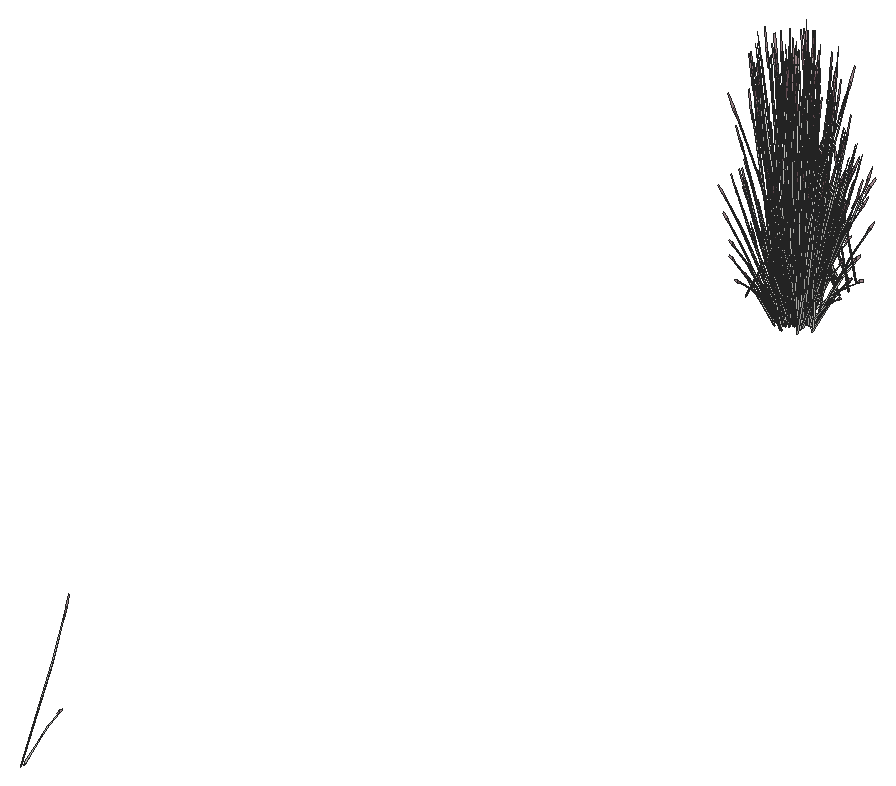
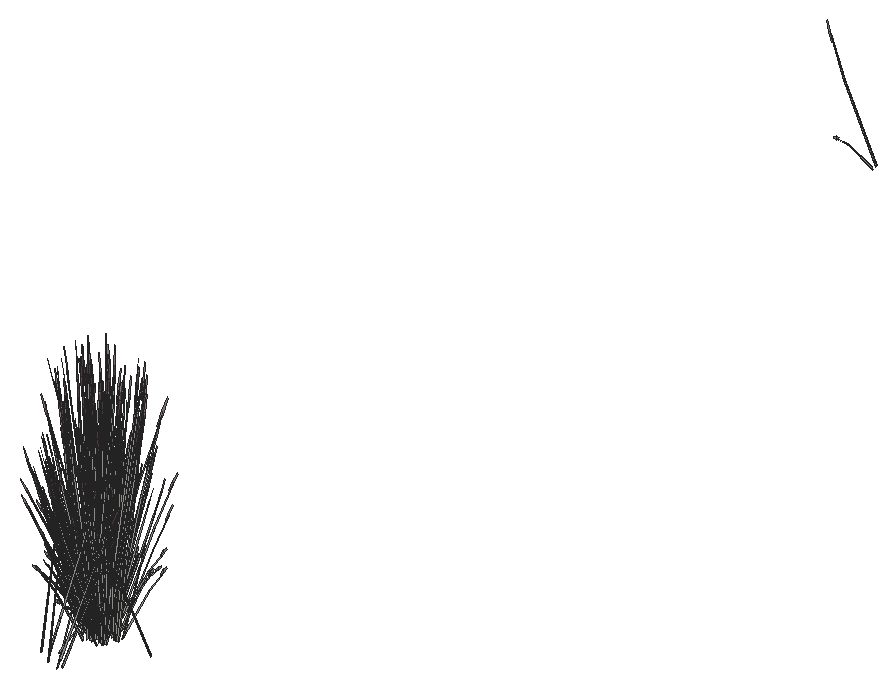
# SketchUp Ruby script. Lengths in inches.
U = 1.inch
M = Sketchup.active_model
def pt(a) = Geom::Point3d.new(a.map { |v| v * U })
def face(e, loops, mat)
  f = e.add_face(loops[0].map { |a| pt(a) })
  loops[1..].each { |l| e.add_face(l.map { |a| pt(a) }).erase! }
  f.material = f.back_material = mat if mat
  f
end
# faces: each face lists its corners as indices into pts; further lists are holes
def faces(e, pts, list, mat = nil) = list.each { |f| face(e, (f[0].is_a?(Array) ? f : [f]).map { |l| l.map { |i| pts[i] } }, mat) }
# xy, xz, yz: faces in a plane at the given z, y or x. An outline is a flat list of corners, or four numbers for a rectangle; further outlines are holes
def ring(l) = l.size == 4 ? [[l[0], l[1]], [l[2], l[1]], [l[2], l[3]], [l[0], l[3]]] : l.each_slice(2).to_a
def flat(e, list, mat, &to3) = list.each { |f| face(e, (f[0].is_a?(Array) ? f : [f]).map { |l| ring(l).map { |u, v| to3.(u, v) } }, mat) }
def xy(e, z, list, mat = nil) = flat(e, list, mat) { |x, y| [x, y, z] }
def xz(e, y, list, mat = nil) = flat(e, list, mat) { |x, z| [x, y, z] }
def yz(e, x, list, mat = nil) = flat(e, list, mat) { |y, z| [x, y, z] }
def lines(e, pts, list) = list.each { |a, b| e.add_line(pt(pts[a]), pt(pts[b])) }
# prism: a flat outline (further loops are holes) pulled along v
def prism(e, loops, v, mat = nil)
  f = face(e, loops, mat); d = Geom::Vector3d.new(v.map { |x| x * U })
  f.pushpull(f.normal.samedirection?(d) ? d.length : -d.length)
end
def box(e, o, s, mat = nil) = prism(e, [[o, [o[0] + s[0], o[1], o[2]], [o[0] + s[0], o[1] + s[1], o[2]], [o[0], o[1] + s[1], o[2]]]], [0, 0, s[2]], mat)
def at(x, y, z, deg = 0) = Geom::Transformation.translation(pt([x, y, z])) * Geom::Transformation.rotation(ORIGIN, Z_AXIS, deg.degrees)
def axes(o, x, y, z) = Geom::Transformation.new([*x, 0, *y, 0, *z, 0, *pt(o).to_a, 1])
def part(name) = M.definitions.add(name)
# library, detail: a bought-in or finely detailed component or shape, given as its bounding box
def library(name, o, s) = part(name).tap { |d| box(d.entities, o, s) }
def detail(e, o, s) = box(e.add_group.entities, o, s)
def put(e, d, t, mat = nil) = e.add_instance(d, t).tap { |i| i.material = mat if mat }
def group(e, t, mat = nil) = e.add_group.tap { |g| g.transformation = t; g.material = mat if mat }.entities
root = M.entities
M.materials.add("LightPink_Translucent").color = [144, 107, 117]
M.materials["LightPink_Translucent"].alpha = 0.75
c1 = part("blade")
p = [[2.15,0.21,22],[0,0.17,0],[0.09,0.45,0],[2.18,0.31,22],[2.29,0.31,22],[0.38,0.45,0],
  [2.48,0.24,33],[2.49,0.24,33],[2.48,0.22,33]]
faces(c1.entities,p,[[0,1,2,3],[4,5,2,3],[6,3,4,7],[8,0,3,6]])
c2 = part("seeds")
p = [[0.3,-0.1,1.38],[-0.01,-0.03,1.59],[-0.01,-0.03,0.03],[0.14,-0.07,-0.07],[0.29,-0.03,3],[0.15,0.01,3.11]]
faces(c2.entities,p,[[0,1,2,3],[1,0,4,5]],"LightPink_Translucent")
c3 = part("blade with seeds")
put(c3.entities,c1,at(0,0,0))
put(c3.entities,c2,axes([2.4,0.25,30.99],[1.5799,-0.05474,1.17369],[-0.12525,1.92788,0.29478],[-0.07173,-0.02425,1.56792]))
put(root,c3,axes([505.97,212.85,4.17],[0.36264,0.49684,-0.71045],[-0.74649,0.27689,0.08574],[0.0848,0.24006,1.00501]))
put(root,c3,axes([505.43,214.1,3.91],[0.09631,0.0984,1.74944],[0.77725,0.03866,-0.27667],[0.07816,0.217,0.14031]))
put(root,c3,axes([507.97,440.58,3.07],[0.17368,0.19618,1.71376],[-0.80256,0.16516,0.13857],[-0.18139,-0.30799,0.73262]))
put(root,c3,axes([509.3,439.28,3.91],[-0.11621,-0.08567,1.74944],[-0.77555,0.05431,-0.27667],[-0.12378,-0.20491,0.14031]))
put(root,c3,axes([511.1,440.3,1.78],[-0.21597,0.12368,1.43002],[-0.64681,-0.21647,-0.30754],[0.1199,-0.26922,0.61141]))
put(root,c3,axes([510.11,440.73,4.17],[-0.36264,-0.49684,-0.71045],[0.74649,-0.27689,0.08574],[-0.0848,-0.24006,1.00501]))
put(root,c3,axes([507.75,440.0625,1.78],[-0.04601,0.19989,1.43002],[-0.67263,0.16733,-0.30754],[-0.15723,-0.25836,0.61141]))
put(root,c3,axes([509.49,439.625,0.6875],[-0.12744,0.02202,1.76342],[-0.70477,-0.24781,-0.26939],[0.01183,-0.2067,0.30037]))
put(root,c3,axes([511.625,441.21,4.17],[0.01977,-0.56521,-0.71045],[0.83252,0.03796,0.08574],[0.08786,-0.23945,1.00501]))
put(root,c3,axes([512.78,440.33,3.91],[-0.00733,-0.12161,1.74944],[-0.61946,-0.35147,-0.27667],[0.09577,-0.21306,0.14031]))
put(root,c3,axes([510.18,440.31,3.72],[0.22906,-0.4699,-0.35414],[0.66828,0.13705,0.4572],[-0.06128,-0.18919,0.87481]))
put(root,c3,axes([510.6875,440.93,3.07],[-0.14147,0.21002,1.71376],[-0.59349,-0.43464,0.13857],[0.26773,-0.27089,0.73262]))
put(root,c3,axes([512.62,439.89,3.9],[-0.07716,0.04667,1.77383],[-0.75601,-0.15746,-0.16761],[-0.02737,-0.20368,0.31391]))
put(root,c3,axes([509.84,440.63,3.875],[-0.7469,-0.15318,-0.51099],[0.25601,-0.52518,-0.3958],[-0.06849,-0.21144,0.97773]))
put(root,c3,axes([510.3,439.3125,1.96],[0.09747,0.35631,1.1486],[-0.54071,-0.19735,0.84392],[0.05818,-0.18244,0.25299]))
put(root,c3,axes([511.45,441.03,3.875],[-0.54391,-0.41056,-0.51099],[0.57458,-0.35956,-0.3958],[0.08276,-0.2086,0.97773]))
put(root,c3,axes([508.5,439,3.9],[-0.01417,0.07324,1.77383],[-0.6991,0.2658,-0.16761],[-0.20573,-0.13587,0.31391]))
put(root,c3,axes([508.35,440.3,4.29],[0.84639,-0.15705,0.53763],[0.14689,0.61608,0.4433],[-0.19906,-0.18157,1.11249]))
put(root,c3,axes([510.26,440.41,3.93],[0.74868,0.15974,0.48003],[-0.25601,0.52518,0.3958],[-0.04499,-0.20653,0.9933]))
put(root,c3,axes([510.48,440.6,4.23],[-0.74352,0.28449,-0.1216],[-0.36538,-0.50492,-0.67495],[-0.0981,-0.21277,1.02557]))
put(root,c3,axes([512.02,441.24,4.23],[-0.83505,-0.03027,-0.1216],[0.02282,-0.57322,-0.67495],[0.05801,-0.22077,1.02557]))
put(root,c3,axes([511.97,440.875,3.72],[0.5141,-0.32171,-0.35414],[0.48666,0.36734,0.4572],[0.07405,-0.18664,0.87481]))
put(root,c3,axes([507.52,439.74,1.96],[0.39634,0.21267,1.1486],[-0.57721,0.12784,0.84392],[-0.1235,-0.16344,0.25299]))
put(root,c3,axes([510.46,440.375,3.92],[0.55987,-0.20767,0.0643],[0.27403,0.37869,0.50621],[-0.05407,-0.16693,0.77189]))
put(root,c3,axes([508.26,440.48,3.72],[-0.11735,-0.49217,-0.35414],[0.67083,-0.12996,0.4572],[-0.18018,-0.14104,0.87481]))
put(root,c3,axes([508.55,440.43,3.92],[0.34533,-0.38816,0.0643],[0.49176,0.22599,0.50621],[-0.15898,-0.12445,0.77189]))
put(root,c3,axes([507.21,440.38,0.6875],[-0.0736,0.08049,1.76342],[-0.74378,0.17355,-0.26939],[-0.17968,-0.15788,0.30037]))
put(root,c3,axes([508.4375,442.59,1.29],[-0.31203,-0.62659,-0.69835],[0.89884,-0.22566,-0.18329],[-0.03449,-0.21218,1.54149]))
put(root,c3,axes([512.61,440.68,0.6875],[-0.11372,-0.04814,1.76342],[-0.29211,-0.53779,-0.26939],[0.19706,-0.14594,0.30037]))
put(root,c3,axes([510.26,440.8,4.24],[-0.22906,0.4699,0.35414],[-0.66828,-0.13705,-0.4572],[-0.06128,-0.18919,0.87481]))
put(root,c3,axes([511.96,441,3.93],[0.54105,0.41691,0.48003],[-0.57458,0.35956,0.3958],[0.0998,-0.1956,0.9933]))
put(root,c3,axes([512.16,441.04,3.92],[0.62439,0.02847,0.0643],[-0.01712,0.42991,0.50621],[0.06534,-0.16468,0.77189]))
put(root,c3,axes([511.7,441.33,4.24],[-0.5141,0.32171,0.35414],[-0.48666,-0.36734,-0.4572],[0.07405,-0.18664,0.87481]))
put(root,c3,axes([512.6,442.2,4.17],[0.39688,-0.48213,-0.71045],[0.69548,0.34264,0.08574],[0.23697,-0.17468,1.00501]))
put(root,c3,axes([508.3125,440.79,1.57],[-0.47504,-0.61229,0],[0.79476,-0.34146,-0.51607],[0.18101,-0.07777,1.63711]))
put(root,c3,axes([512.58,441.97,3.875],[-0.19519,-0.55794,-0.51099],[0.73919,-0.0976,-0.3958],[0.21183,-0.14986,0.97773]))
put(root,c3,axes([509.36,440.05,1.32],[-0.52505,0.35054,-0.03893],[-0.48109,-0.38392,-0.17649],[-0.03387,-0.10878,0.58215]))
put(root,c3,axes([512.93,442.37,4.23],[-0.70283,-0.33692,-0.1216],[0.40491,-0.48793,-0.67495],[0.19857,-0.16961,1.02557]))
put(root,c3,axes([510.03,444.21,2.52],[0.65659,0.2464,1.51261],[-0.64324,0.53082,0.59816],[-0.28812,-0.31461,1.26806]))
put(root,c3,axes([508.65,440.88,4.24],[0.11735,0.49217,0.35414],[-0.67083,0.12996,-0.4572],[-0.18018,-0.14104,0.87481]))
put(root,c3,axes([506.6,442.51,1.21],[0,-0.61104,-0.49651],[0.85008,0,0],[0,-0.13917,1.57504]))
put(root,c3,axes([508.96,440.7,1.21],[0.7111,-0.30552,-0.49651],[0.42504,0.54784,0],[0.16196,-0.06958,1.57504]))
put(root,c3,axes([513.18,441.75,1.78],[-0.27143,-0.0181,1.43002],[-0.27808,-0.48551,-0.30754],[0.33346,-0.13735,0.61141]))
put(root,c3,axes([514.66,442.22,3.9],[-0.09924,-0.00464,1.77383],[-0.4121,-0.49725,-0.16761],[0.1655,-0.1635,0.31391]))
put(root,c3,axes([509.8,441.95,1.25],[0.51177,-0.45928,-0.62353],[0.63575,0.41646,-0.16365],[0.20507,-0.11457,1.37633]))
put(root,c3,axes([513.49,440.86,1.96],[-0.25308,0.31105,1.1486],[-0.21753,-0.4179,0.84392],[0.20902,-0.10472,0.25299]))
put(root,c3,axes([513.13,442.03,3.72],[0.66138,-0.08733,-0.35414],[0.17464,0.49921,0.4572],[0.18953,-0.13408,0.87481]))
put(root,c3,axes([508.91,442.76,1.4],[0.36864,-0.55059,-0.44739],[0.76598,0.26498,0.21531],[0,-0.12692,1.43643]))
put(root,c3,axes([509.25,442.48,1.86],[-0.08854,-0.69723,-0.29095],[0.92215,-0.04216,-0.50002],[0.16238,-0.09287,1.59708]))
put(root,c3,axes([506.96,442.52,1.22],[0.53038,-0.38124,-0.30978],[0.53038,0.38124,0.30978],[0,-0.1228,1.38974]))
put(root,c3,axes([506.75,440.69,1.32],[-0.21918,0.49894,-0.03893],[-0.6746,-0.15348,-0.17649],[-0.10242,-0.08161,0.58215]))
put(root,c3,axes([512.59,442.32,4.24],[-0.66138,0.08733,0.35414],[-0.17464,-0.49921,-0.4572],[0.18953,-0.13408,0.87481]))
put(root,c3,axes([508.82,443.21,1.86],[-0.85568,-0.29155,-0.29095],[0.41201,-0.61537,-0.50002],[-0.02689,-0.15109,1.59708]))
put(root,c3,axes([506.38,442.97,1.57],[-0.95008,0,0],[0,-0.68292,-0.51607],[0,-0.15554,1.63711]))
put(root,c3,axes([509.125,440.9375,1.22],[0.70886,0.15119,-0.30978],[-0.17848,0.53243,0.30978],[0.1429,-0.0614,1.38974]))
put(root,c3,axes([513.19,442.25,3.92],[0.52161,0.25698,0.0643],[-0.30368,0.36595,0.50621],[0.16723,-0.11831,0.77189]))
put(root,c3,axes([513.04,442.14,3.93],[0.18844,0.56237,0.48003],[-0.73919,0.0976,0.3958],[0.21785,-0.13226,0.9933]))
put(root,c3,axes([515.04,442.82,3.91],[0.10543,-0.09307,1.74944],[-0.13495,-0.57092,-0.27667],[0.26455,-0.10825,0.14031]))
put(root,c3,axes([507.12,442.79,1.52],[-0.70674,0.51372,0.30756],[-0.70717,-0.50832,-0.36492],[-0.02468,-0.14589,1.64885]))
put(root,c3,axes([509.37,443.03,1.625],[0.8561,0.29616,0.24065],[-0.41201,0.61537,0.50002],[0,-0.14185,1.60543]))
put(root,c3,axes([509.03,443.86,1.63],[0.20138,-0.72405,-0.23429],[0.95485,0.12621,0.51271],[-0.16685,-0.09999,1.5644]))
put(root,c3,axes([509.09,442.62,1.91],[-0.82508,0.03772,0.44739],[-0.07462,-0.62614,-0.21531],[0.14771,-0.06346,1.43643]))
put(root,c3,axes([506.96,443.07,1.67],[0,0.61104,0.49651],[-0.85008,0,0],[0,-0.13917,1.57504]))
put(root,c3,axes([512.96,443.69,4.23],[-0.38229,-0.5533,-0.1216],[0.6785,-0.2719,-0.67495],[0.28593,-0.073,1.02557]))
put(root,c3,axes([512.93,443.21,3.875],[0.20584,-0.55581,-0.51099],[0.70573,0.19051,-0.3958],[0.28414,-0.05097,0.97773]))
put(root,c3,axes([511.8125,440.95,1.57],[0.47504,-0.61229,0],[0.79476,0.34146,-0.51607],[0.18101,0.07777,1.63711]))
put(root,c3,axes([508.97,443.57,1.4],[-0.45644,-0.51287,-0.44739],[0.69137,-0.36116,0.21531],[-0.14771,-0.06346,1.43643]))
put(root,c3,axes([509.0625,442.84,1.55],[0.33034,0.68327,0.45755],[-0.94388,0.2376,0.17955],[0.01154,-0.12555,1.58856]))
put(root,c3,axes([513.68,443.37,1.17],[-0.48937,0.07333,1.41583],[-0.07789,-0.58369,0.08104],[0.34275,-0.08835,0.80566]))
put(root,c3,axes([514.57,442.85,1.45],[-0.47106,-0.39072,-0.06488],[0.51591,-0.35801,-0.29416],[0.14618,-0.02521,0.97024]))
put(root,c3,axes([508.9,443.38,1.91],[-0.36864,0.55059,0.44739],[-0.76598,-0.26498,-0.21531],[0,-0.12692,1.43643]))
put(root,c3,axes([510.25,442.9,1.4],[0,-0.70701,0],[0.95008,0,0],[0,0,1.79456]))
put(root,c3,axes([511.4,441.27,1.67],[-0.7111,-0.30552,0.49651],[0.42504,-0.54784,0],[0.16196,0.06958,1.57504]))
put(root,c3,axes([512.79,443.41,4.17],[0.66765,-0.26986,-0.71045],[0.37208,0.55551,0.08574],[0.32259,-0.0631,1.00501]))
put(root,c3,axes([509.8,442.45,1.55],[-0.62999,0.55453,0.45755],[-0.74845,-0.4895,0.17955],[0.15188,-0.05534,1.58856]))
put(root,c3,axes([510.49,443.45,1.49],[-0.70674,-0.52593,-0.06131],[0.70717,-0.52625,0],[-0.02468,-0.01837,1.75571]))
put(root,c3,axes([508.71,441.54,1.67],[-0.21949,0.60727,0.17642],[-0.8032,-0.17185,0.35086],[0.13875,-0.00296,1.60407]))
put(root,c3,axes([512.7,443.52,4.24],[-0.63144,-0.17046,0.35414],[0.18417,-0.49731,-0.4572],[0.25423,-0.0456,0.87481]))
put(root,c3,axes([508.375,442.03,0.79],[-0.74787,0.24464,1.28929],[-0.23804,-0.70192,0.50096],[0.45924,0.01168,1.46642]))
put(root,c3,axes([510.38,442.22,1.81],[0.14658,-0.54532,0.1448],[0.71613,0.09466,-0.41347],[0.13033,0.05599,1.26744]))
put(root,c3,axes([509.15,443.51,1.55],[0.96033,0.12874,0.45755],[-0.19544,0.7271,0.17955],[-0.14034,-0.07021,1.58856]))
put(root,c3,axes([514.22,442.98,0.6875],[-0.03971,-0.09277,1.76342],[0.27541,-0.54264,-0.26939],[0.27782,-0.00781,0.30037]))
put(root,c3,axes([510.08,442.36,1.91],[-0.45644,-0.51287,0.44739],[0.69137,-0.36116,-0.21531],[0.14771,0.06346,1.43643]))
put(root,c3,axes([507.72,444.7,1.22],[-0.17848,-0.53243,-0.30978],[0.70886,-0.15119,0.30978],[-0.1429,-0.0614,1.38974]))
put(root,c3,axes([508.63,444.67,1.67],[0.81646,-0.16218,0.17642],[0.20161,0.60355,0.35086],[-0.07282,-0.08794,1.60407]))
put(root,c3,axes([510.3125,442.39,1.86],[0.76714,-0.40567,-0.29095],[0.51013,0.57321,-0.50002],[0.18927,0.05821,1.59708]))
put(root,c3,axes([513.36,443.46,3.72],[0.63144,0.17046,-0.35414],[-0.18417,0.49731,0.4572],[0.25423,-0.0456,0.87481]))
put(root,c3,axes([507.52,444.93,1.21],[-0.7111,-0.30552,-0.49651],[0.42504,-0.54784,0],[-0.16196,-0.06958,1.57504]))
put(root,c3,axes([512.24,441.32,1.21],[0.7111,0.30552,-0.49651],[-0.42504,0.54784,0],[0.16196,0.06958,1.57504]))
put(root,c3,axes([510.9,443.06,1.4],[0.85008,0,0],[0,0.63259,0],[0,0,1.78407]))
put(root,c3,axes([509.45,443.85,1.86],[-0.76714,0.40567,-0.29095],[-0.51013,-0.57321,-0.50002],[-0.18927,-0.05821,1.59708]))
put(root,c3,axes([511.14,441.57,1.67],[-0.81646,0.16218,0.17642],[-0.20161,-0.60355,0.35086],[0.07282,0.08794,1.60407]))
put(root,c3,axes([511.64,442.85,3.07],[-0.31515,0.01384,1.71376],[0.20907,-0.5998,0.13857],[0.44912,0.0371,0.73262]))
put(root,c3,axes([512.05,441.54,1.22],[0.17848,0.53243,-0.30978],[-0.70886,0.15119,0.30978],[0.1429,0.0614,1.38974]))
put(root,c3,axes([513.27,443.67,3.92],[0.27906,0.41663,0.0643],[-0.50888,0.20393,0.50621],[0.22432,-0.04024,0.77189]))
put(root,c3,axes([510.62,442.74,1.57],[-0.96033,-0.12874,0.49198],[0.19544,-0.7271,0.19306],[0.14034,0.07021,1.70813]))
put(root,c3,axes([513.21,443.52,3.93],[-0.21466,0.55714,0.48003],[-0.70573,-0.19051,0.3958],[0.27753,-0.03348,0.9933]))
put(root,c3,axes([509.86,444.53,1.4],[-0.24791,-0.5268,0],[0.70791,-0.18448,0],[0,0,1.54371]))
put(root,c3,axes([509.38,444.03,1.81],[-0.14658,0.54532,0.1448],[-0.71613,-0.09466,-0.41347],[-0.13033,-0.05599,1.26744]))
put(root,c3,axes([510.78,444.46,1.38],[0.79769,-0.20732,-0.19198],[0.2803,0.59721,0.00008],[0.08805,-0.02292,1.73897]))
put(root,c3,axes([511.06,444.71,1.67],[0.21949,-0.60727,0.17642],[0.8032,0.17185,0.35086],[-0.13875,0.00296,1.60407]))
put(root,c3,axes([510.875,443.33,1.41],[0.53038,0.39469,0],[-0.53038,0.39469,0],[0,0,1.69266]))
put(root,c3,axes([512.3125,443.16,1.67],[-0.59697,-0.44509,0.17642],[0.60159,-0.4317,0.35086],[-0.06593,0.0909,1.60407]))
put(root,c3,axes([511.21,442.49,1.25],[0.79037,0.10018,-0.62353],[-0.16679,0.61794,-0.16365],[0.23587,0.07488,1.37633]))
put(root,c3,axes([514.7,443.56,1.96],[-0.46945,0.10088,1.1486],[0.22097,-0.4169,0.84392],[0.24904,0.02853,0.25299]))
put(root,c3,axes([509.68,444.77,1.39],[-0.76598,-0.27433,0],[0.36864,-0.57001,0],[0,0,1.62707]))
put(root,c3,axes([510.32,444.04,1.66],[-0.74193,-0.49181,-0.25192],[0.6243,-0.55226,0.5513],[-0.19979,0.05753,1.68216]))
put(root,c3,axes([508.36,444.98,1.67],[0.7111,0.30552,0.49651],[-0.42504,0.54784,0],[-0.16196,-0.06958,1.57504]))
put(root,c3,axes([510.87,442.87,1.91],[0.36864,-0.55059,0.44739],[0.76598,0.26498,-0.21531],[0,0.12692,1.43643]))
put(root,c3,axes([514.48,445.33,3.9],[-0.0687,-0.05349,1.77383],[0.15029,-0.57341,-0.16761],[0.27062,-0.03664,0.31391]))
put(root,c3,axes([510.73,443.18,1.48],[0,0.70667,-0.05637],[-0.95008,0,0],[0,0.02221,1.79368]))
put(root,c3,axes([510.8,442.68,1.4],[0.45644,0.51287,-0.44739],[-0.69137,0.36116,0.21531],[0.14771,0.06346,1.43643]))
put(root,c3,axes([513.88,444.85,3.12],[-0.14542,-0.51365,-0.03492],[0.68734,-0.11809,-0.15832],[0.14353,0.03256,0.52218]))
put(root,c3,axes([507.95,445.3,1.57],[-0.47504,0.61229,0],[-0.79476,-0.34146,-0.51607],[-0.18101,-0.07777,1.63711]))
put(root,c3,axes([512.1,444.83,4.23],[0.04068,-0.62141,-0.1216],[0.77029,0.01698,-0.67495],[0.29667,0.04317,1.02557]))
put(root,c3,axes([512.8,443.17,1.67],[0,-0.61104,0.49651],[0.85008,0,0],[0,0.13917,1.57504]))
put(root,c3,axes([510.67,443.63,1.91],[0.82508,-0.03772,0.44739],[0.07462,0.62614,-0.21531],[-0.14771,0.06346,1.43643]))
put(root,c3,axes([511.19,442.99,1.81],[0.70791,-0.1782,0.1448],[0.24791,0.50885,-0.41347],[0,0.11199,1.26744]))
put(root,c3,axes([511.98,444.59,4.24],[-0.43232,-0.38257,0.35414],[0.49364,-0.36215,-0.4572],[0.25081,0.0551,0.87481]))
put(root,c3,axes([509.94,443.94,1.4],[-0.82508,0.03772,-0.44739],[-0.07462,-0.62614,0.21531],[-0.14771,0.06346,1.43643]))
put(root,c3,axes([497.11,444.23,1.78],[-0.18299,-0.15028,1.43002],[0.23809,-0.49714,-0.30754],[0.37023,0.06735,0.61141]))
put(root,c3,axes([513.82,444.23,1.78],[-0.18299,-0.15028,1.43002],[0.23809,-0.49714,-0.30754],[0.37023,0.06735,0.61141]))
put(root,c3,axes([510.55,444.78,1.4],[0.76598,0.27433,0],[-0.36864,0.57001,0],[0,0,1.74954]))
put(root,c3,axes([512.77,444.46,3.91],[0.16299,-0.01033,1.74944],[0.44707,-0.47471,-0.27667],[0.28992,0.06266,0.14031]))
put(root,c3,axes([510.85,445.39,1.39],[-0.46912,-0.61443,-0.05142],[0.79476,-0.34146,0.51607],[-0.19584,0.0585,1.6363]))
put(root,c3,axes([510.6875,443.9,1.81],[0.56134,0.36712,0.1448],[-0.46823,0.41419,-0.41347],[-0.13033,0.05599,1.26744]))
put(root,c3,axes([512.14,444.54,4.17],[0.75952,0.01471,-0.71045],[-0.05101,0.61953,0.08574],[0.32177,0.06538,1.00501]))
put(root,c3,axes([511.29,445.03,1.67],[0.7111,-0.30552,0.49651],[0.42504,0.54784,0],[-0.16196,0.06958,1.57504]))
put(root,c3,axes([510.27,444.55,1.48],[0.33034,0.70197,-0.06012],[-0.94388,0.24598,0],[0.01154,0.02451,1.72173]))
put(root,c3,axes([510.64,445.31,1.22],[-0.70886,-0.15119,-0.30978],[0.17848,-0.53243,0.30978],[-0.1429,0.0614,1.38974]))
put(root,c3,axes([506.71,443.81,4.24],[0.66138,-0.08733,0.35414],[0.17464,0.49921,-0.4572],[-0.18953,0.13408,0.87481]))
put(root,c3,axes([513.38,443.28,1.57],[0.95008,0,0],[0,0.68292,-0.51607],[0,0.15554,1.63711]))
put(root,c3,axes([513,443.63,1.39],[-0.94962,-0.00489,-0.04976],[0,-0.68292,0.49943],[-0.02984,0.15546,1.58352]))
put(root,c3,axes([510.95,443.03,1.86],[0.85568,0.29155,-0.29095],[-0.41201,0.61537,-0.50002],[0.02689,0.15109,1.59708]))
put(root,c3,axes([512.6,444.79,3.72],[0.43232,0.38257,-0.35414],[-0.49364,0.36215,0.4572],[0.25081,0.0551,0.87481]))
put(root,c3,axes([512.8,443.73,1.22],[-0.53038,0.38124,-0.30978],[-0.53038,-0.38124,0.30978],[0,0.1228,1.38974]))
put(root,c3,axes([510.52,443.77,1.86],[0.08854,0.69723,-0.29095],[-0.92215,0.04216,-0.50002],[-0.16238,0.09287,1.59708]))
put(root,c3,axes([512.375,444.9375,3.92],[-0.03826,0.46465,0.0643],[-0.57772,-0.01274,0.50621],[0.2213,0.04862,0.77189]))
put(root,c3,axes([510.86,443.49,1.4],[-0.36864,0.55059,-0.44739],[-0.76598,-0.26498,0.21531],[0,0.12692,1.43643]))
put(root,c3,axes([512.43,444.79,3.93],[-0.56024,0.40262,0.48003],[-0.48318,-0.42758,0.3958],[0.26285,0.07427,0.9933]))
put(root,c3,axes([505.21,445.23,4.84],[0.67048,0.16311,-0.06488],[-0.20625,0.50201,-0.29416],[-0.10966,0.07622,0.97024]))
put(root,c3,axes([509.96,444.3,1.25],[-0.51177,0.45928,-0.62353],[-0.63575,-0.41646,-0.16365],[-0.20507,0.11457,1.37633]))
put(root,c3,axes([510.65,445.26,4.24],[-0.11735,-0.49217,0.35414],[0.67083,-0.12996,-0.4572],[0.18018,0.14104,0.87481]))
put(root,c3,axes([510.875,445.07,1.52],[0.95122,0.19861,0.30756],[-0.23797,0.7099,-0.36492],[-0.15744,0.08885,1.64885]))
put(root,c3,axes([510.81,445.55,1.21],[-0.7111,0.30552,-0.49651],[-0.42504,-0.54784,0],[-0.16196,0.06958,1.57504]))
put(root,c3,axes([513.17,443.74,1.21],[0,0.61104,-0.49651],[-0.85008,0,0],[0,0.13917,1.57504]))
put(root,c3,axes([511.04,443.81,3.07],[-0.28223,-0.10528,1.71376],[0.58406,-0.44165,0.13857],[0.36402,0.19924,0.73262]))
put(root,c3,axes([511.1,442.42,3.67],[-0.65655,-0.31748,1.38283],[0.69326,-0.49431,0.59665],[0.21183,0.29789,1.33663]))
put(root,c3,axes([506.37,443.76,4.23],[0.70283,0.33692,-0.1216],[-0.40491,0.48793,-0.67495],[-0.19857,0.16961,1.02557]))
put(root,c3,axes([512.09,445.01,1.96],[-0.4278,-0.1757,1.1486],[0.5524,-0.17852,0.84392],[0.14899,0.15122,0.25299]))
put(root,c3,axes([510.59,445.51,4.23],[0.45276,-0.52302,-0.1216],[0.65568,0.30132,-0.67495],[0.22792,0.14777,1.02557]))
put(root,c3,axes([507.6,444.8,4.24],[0.5141,-0.32171,0.35414],[0.48666,0.36734,-0.4572],[-0.07405,0.18664,0.87481]))
put(root,c3,axes([511.45,445.46,1.57],[0.47504,0.61229,0],[-0.79476,0.34146,-0.51607],[-0.18101,0.07777,1.63711]))
put(root,c3,axes([509.99,445.94,3.9],[0.00225,-0.07398,1.77383],[0.65113,-0.32638,-0.16761],[0.22617,0.1165,0.31391]))
put(root,c3,axes([512.21,445.66,0.6875],[0.05536,-0.08822,1.76342],[0.69692,-0.25981,-0.26939],[0.21129,0.13447,0.30037]))
put(root,c3,axes([511.05,443.03,2.03],[-0.02076,-0.57531,1.41272],[0.93937,0.14913,0.59816],[-0.22217,0.31481,1.3335]))
put(root,c3,axes([511.29,443.66,1.29],[0.2786,0.55945,-0.69212],[-0.80253,0.20149,-0.18165],[0.03079,0.18945,1.52773]))
put(root,c3,axes([507.14,445.1,3.92],[-0.62439,-0.02847,0.0643],[0.01712,-0.42991,0.50621],[-0.06534,0.16468,0.77189]))
put(root,c3,axes([507.33,445.14,3.93],[-0.54105,-0.41691,0.48003],[0.57458,-0.35956,0.3958],[-0.0998,0.1956,0.9933]))
put(root,c3,axes([511.12,445.25,3.875],[0.74975,-0.14525,-0.51099],[0.13115,0.55007,-0.3958],[0.20138,0.15763,0.97773]))
put(root,c3,axes([509.04,445.33,4.24],[0.22906,-0.4699,0.35414],[0.66828,0.13705,-0.4572],[0.06128,0.18919,0.87481]))
put(root,c3,axes([512.16,445.81,1.86],[-0.48723,-0.01916,1.0506],[0.32177,-0.40701,0.58006],[0.19248,0.1446,0.8241]))
put(root,c3,axes([510.75,445.7,3.92],[-0.34533,0.38816,0.0643],[-0.49176,-0.22599,0.50621],[0.15898,0.12445,0.77189]))
put(root,c3,axes([509.94,447.01,4.84],[0.52505,-0.35054,-0.06488],[0.48109,0.38392,-0.29416],[0.03387,0.10878,0.97024]))
put(root,c3,axes([510.9,445.59,3.93],[-0.75571,0.14023,0.48003],[-0.13115,-0.55007,0.3958],[0.17773,0.16212,0.9933]))
put(root,c3,axes([510.57,444.82,1.78],[0.01341,-0.20255,1.43002],[0.64074,-0.22625,-0.30754],[0.1978,0.24243,0.61141]))
put(root,c3,axes([508.84,445.76,3.92],[-0.55987,0.20767,0.0643],[-0.27403,-0.37869,0.50621],[0.05407,0.16693,0.77189]))
put(root,c3,axes([507.33,445.26,3.72],[-0.5141,0.32171,-0.35414],[-0.48666,-0.36734,0.4572],[-0.07405,0.18664,0.87481]))
put(root,c3,axes([507.27,444.89,4.59],[0.83505,0.03027,-0.13498],[-0.02282,0.57322,-0.74919],[-0.05801,0.22077,1.13838]))
put(root,c3,axes([508.82,445.53,4.23],[0.74352,-0.28449,-0.1216],[0.36538,0.50492,-0.67495],[0.0981,0.21277,1.02557]))
put(root,c3,axes([509.03,445.72,4.26],[-0.74868,-0.15974,0.53283],[0.25601,-0.52518,0.43934],[0.04499,0.20653,1.10256]))
put(root,c3,axes([507.66,446.51,1.96],[-0.01966,-0.36332,1.1486],[0.49135,0.25914,0.84392],[-0.09663,0.17317,0.25299]))
put(root,c3,axes([508.95,445.64,0.6875],[0.12297,-0.03325,1.76342],[0.73967,0.18301,-0.26939],[0.02163,0.20626,0.30037]))
put(root,c3,axes([507.84,445.11,4.2],[0.54391,0.41056,-0.5672],[-0.57458,0.35956,-0.43934],[-0.08276,0.2086,1.08528]))
put(root,c3,axes([507.25,445.73,2.02],[0.69024,-0.1082,0.06507],[0.15868,0.43593,-0.86304],[-0.04376,0.22067,0.7736]))
put(root,c3,axes([509.46,445.51,3.875],[0.7469,0.15318,-0.51099],[-0.25601,0.52518,-0.3958],[0.06849,0.21144,0.97773]))
put(root,c3,axes([509.88,444.42,3.07],[-0.17368,-0.19618,1.71376],[0.80256,-0.16516,0.13857],[0.18139,0.30799,0.73262]))
put(root,c3,axes([509.12,445.83,3.72],[-0.22906,0.4699,-0.35414],[-0.66828,-0.13705,0.4572],[0.06128,0.18919,0.87481]))
put(root,c3,axes([507.68,444.92,4.53],[-0.01977,0.56521,-0.7886],[-0.83252,-0.03796,0.09517],[-0.08786,0.23945,1.11556]))
put(root,c3,axes([505.5,446.41,3.9],[0.0862,-0.03689,1.77383],[0.71245,0.24539,-0.16761],[-0.01674,0.20431,0.31391]))
put(root,c3,axes([508.46,444.52,3.07],[-0.0186,-0.23452,1.71376],[0.80601,0.15558,0.13857],[-0.04985,0.33422,0.73262]))
put(root,c3,axes([509.1875,445.41,4.17],[0.36264,0.49684,-0.71045],[-0.74649,0.27689,0.08574],[0.0848,0.24006,1.00501]))
put(root,c3,axes([507.09,446.1875,1.78],[0.23977,-0.09639,1.43002],[0.59198,0.29065,-0.30754],[-0.1762,0.25149,0.61141]))
put(root,c3,axes([508.64,446.66,3.91],[0.09631,0.0984,1.74944],[0.77725,0.03866,-0.27667],[0.07816,0.217,0.14031]))
put(root,c3,axes([507.4,445.72,2.56],[0.01669,-0.31544,1.54345],[0.75083,0.16661,0.21329],[-0.06506,0.33618,0.72882]))
put(root,c3,axes([508.09,458.2,3.07],[0.17368,0.19618,1.71376],[-0.80256,0.16516,0.13857],[-0.18139,-0.30799,0.73262]))
put(root,c3,axes([509.41,456.9,3.91],[-0.11621,-0.08567,1.74944],[-0.77555,0.05431,-0.27667],[-0.12378,-0.20491,0.14031]))
put(root,c3,axes([511.21,457.92,1.78],[-0.21597,0.12368,1.43002],[-0.64681,-0.21647,-0.30754],[0.1199,-0.26922,0.61141]))
put(root,c3,axes([510.23,458.35,4.17],[-0.36264,-0.49684,-0.71045],[0.74649,-0.27689,0.08574],[-0.0848,-0.24006,1.00501]))
put(root,c3,axes([507.87,457.68,1.78],[-0.04601,0.19989,1.43002],[-0.67263,0.16733,-0.30754],[-0.15723,-0.25836,0.61141]))
put(root,c3,axes([509.6,457.24,0.6875],[-0.12744,0.02202,1.76342],[-0.70477,-0.24781,-0.26939],[0.01183,-0.2067,0.30037]))
put(root,c3,axes([511.74,458.83,4.17],[0.01977,-0.56521,-0.71045],[0.83252,0.03796,0.08574],[0.08786,-0.23945,1.00501]))
